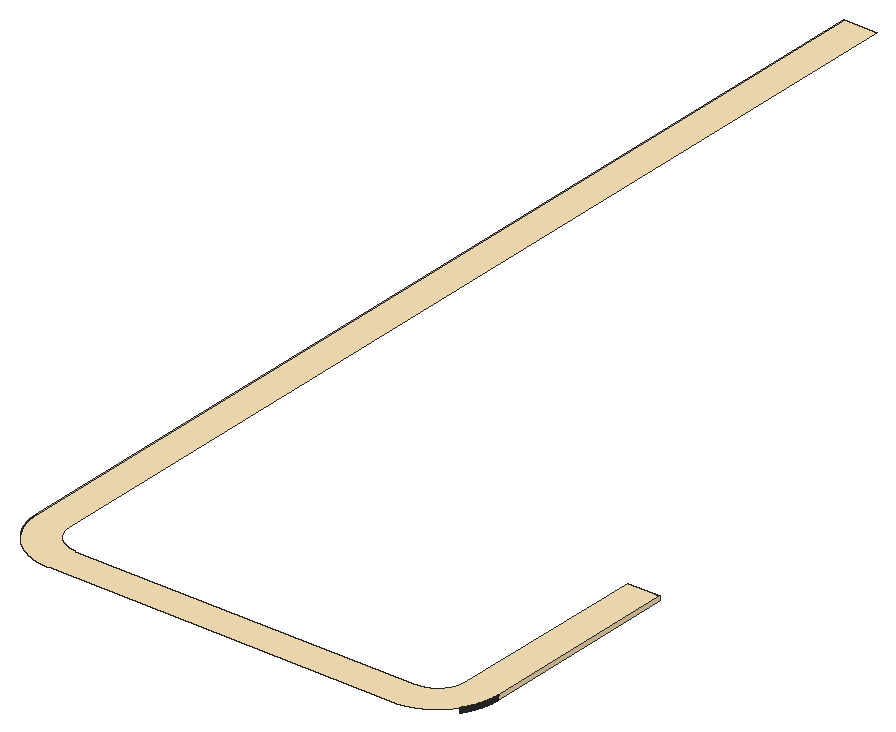
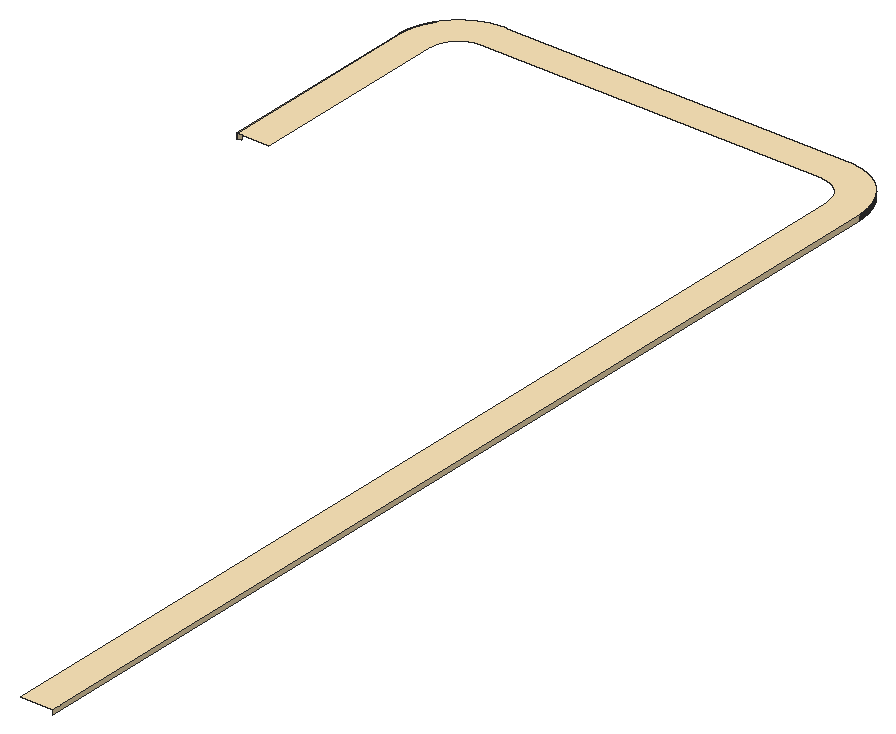
# SketchUp Ruby script. Lengths in inches.
U = 1.inch
M = Sketchup.active_model
def pt(a) = Geom::Point3d.new(a.map { |v| v * U })
def face(e, loops, mat)
  f = e.add_face(loops[0].map { |a| pt(a) })
  loops[1..].each { |l| e.add_face(l.map { |a| pt(a) }).erase! }
  f.material = f.back_material = mat if mat
  f
end
# faces: each face lists its corners as indices into pts; further lists are holes
def faces(e, pts, list, mat = nil) = list.each { |f| face(e, (f[0].is_a?(Array) ? f : [f]).map { |l| l.map { |i| pts[i] } }, mat) }
# xy, xz, yz: faces in a plane at the given z, y or x. An outline is a flat list of corners, or four numbers for a rectangle; further outlines are holes
def ring(l) = l.size == 4 ? [[l[0], l[1]], [l[2], l[1]], [l[2], l[3]], [l[0], l[3]]] : l.each_slice(2).to_a
def flat(e, list, mat, &to3) = list.each { |f| face(e, (f[0].is_a?(Array) ? f : [f]).map { |l| ring(l).map { |u, v| to3.(u, v) } }, mat) }
def xy(e, z, list, mat = nil) = flat(e, list, mat) { |x, y| [x, y, z] }
def xz(e, y, list, mat = nil) = flat(e, list, mat) { |x, z| [x, y, z] }
def yz(e, x, list, mat = nil) = flat(e, list, mat) { |y, z| [x, y, z] }
def lines(e, pts, list) = list.each { |a, b| e.add_line(pt(pts[a]), pt(pts[b])) }
# prism: a flat outline (further loops are holes) pulled along v
def prism(e, loops, v, mat = nil)
  f = face(e, loops, mat); d = Geom::Vector3d.new(v.map { |x| x * U })
  f.pushpull(f.normal.samedirection?(d) ? d.length : -d.length)
end
def box(e, o, s, mat = nil) = prism(e, [[o, [o[0] + s[0], o[1], o[2]], [o[0] + s[0], o[1] + s[1], o[2]], [o[0], o[1] + s[1], o[2]]]], [0, 0, s[2]], mat)
def at(x, y, z, deg = 0) = Geom::Transformation.translation(pt([x, y, z])) * Geom::Transformation.rotation(ORIGIN, Z_AXIS, deg.degrees)
def axes(o, x, y, z) = Geom::Transformation.new([*x, 0, *y, 0, *z, 0, *pt(o).to_a, 1])
def part(name) = M.definitions.add(name)
# library, detail: a bought-in or finely detailed component or shape, given as its bounding box
def library(name, o, s) = part(name).tap { |d| box(d.entities, o, s) }
def detail(e, o, s) = box(e.add_group.entities, o, s)
def put(e, d, t, mat = nil) = e.add_instance(d, t).tap { |i| i.material = mat if mat }
def group(e, t, mat = nil) = e.add_group.tap { |g| g.transformation = t; g.material = mat if mat }.entities
root = M.entities
M.materials.add("1026 AP 7946 SUNNY SIDE UP").color = [254, 231, 186]
xy(root,276,[[[177,213,177.272,213.001,177.545,213.006,177.817,213.013,178.089,213.023,178.361,213.036,178.633,213.051,178.904,213.07,179.176,213.091,179.447,213.115,179.718,213.142,179.988,213.172,180.259,213.205,180.529,213.241,180.798,213.279,181.067,213.32,181.336,213.364,181.604,213.411,181.872,213.461,182.139,213.513,182.406,213.568,182.672,213.626,182.937,213.687,183.202,213.751,183.466,213.817,183.729,213.886,183.992,213.958,184.254,214.032,184.515,214.11,184.775,214.19,185.034,214.273,185.293,214.358,185.551,214.446,185.807,214.537,186.063,214.631,186.318,214.727,186.571,214.826,186.824,214.927,187.075,215.032,187.326,215.138,187.575,215.248,187.823,215.36,188.07,215.474,188.316,215.592,188.561,215.711,188.804,215.834,189.046,215.959,189.286,216.086,189.526,216.216,189.763,216.348,190,216.483,190.235,216.621,190.469,216.761,190.701,216.903,190.931,217.047,191.161,217.195,191.388,217.344,191.614,217.496,191.839,217.65,192.061,217.807,192.282,217.966,192.502,218.127,192.72,218.29,192.936,218.456,193.15,218.624,193.362,218.794,193.573,218.967,193.782,219.141,193.989,219.318,194.194,219.497,194.397,219.678,194.599,219.861,194.798,220.047,194.996,220.234,195.191,220.424,195.385,220.615,195.576,220.809,195.766,221.004,195.953,221.202,196.139,221.401,196.322,221.603,196.503,221.806,196.682,222.011,196.859,222.218,197.033,222.427,197.206,222.638,197.376,222.85,197.544,223.064,197.71,223.28,197.873,223.498,198.034,223.718,198.193,223.939,198.35,224.161,198.504,224.386,198.656,224.612,198.805,224.839,198.953,225.069,199.097,225.299,199.239,225.531,199.379,225.765,199.517,226,199.652,226.237,199.784,226.474,199.914,226.714,200.041,226.954,200.166,227.196,200.289,227.439,200.408,227.684,200.526,227.93,200.64,228.177,200.752,228.425,200.862,228.674,200.968,228.925,201.073,229.176,201.174,229.429,201.273,229.682,201.369,229.937,201.463,230.193,201.554,230.449,201.642,230.707,201.727,230.966,201.81,231.225,201.89,231.485,201.968,231.746,202.042,232.008,202.114,232.271,202.183,232.534,202.249,232.798,202.313,233.063,202.374,233.328,202.432,233.594,202.487,233.861,202.539,234.128,202.589,234.396,202.636,234.664,202.68,234.933,202.721,235.202,202.759,235.471,202.795,235.741,202.828,236.012,202.858,236.282,202.885,236.553,202.909,236.824,202.93,237.096,202.949,237.367,202.964,237.639,202.977,237.911,202.987,238.183,202.994,238.455,202.999,238.728,203,239,203,326,189,326,189,239,188.997,238.749,188.994,238.623,188.989,238.497,188.984,238.372,188.976,238.247,188.968,238.121,188.958,237.996,188.947,237.871,188.934,237.746,188.92,237.621,188.905,237.496,188.889,237.371,188.871,237.247,188.852,237.123,188.832,236.999,188.81,236.875,188.787,236.751,188.763,236.628,188.738,236.505,188.711,236.382,188.683,236.26,188.654,236.138,188.623,236.016,188.591,235.894,188.558,235.773,188.524,235.652,188.488,235.532,188.451,235.412,188.413,235.292,188.373,235.172,188.333,235.054,188.291,234.935,188.247,234.817,188.203,234.7,188.157,234.583,188.11,234.466,188.0625,234.35,188.013,234.234,187.963,234.119,187.911,234.005,187.858,233.891,187.804,233.777,187.749,233.664,187.692,233.552,187.634,233.44,187.576,233.329,187.516,233.219,187.455,233.109,187.392,233,187.329,232.892,187.264,232.784,187.199,232.677,187.132,232.57,187.064,232.464,186.995,232.359,186.925,232.255,186.854,232.151,186.782,232.049,186.634,231.845,186.482,231.645,186.404,231.546,186.326,231.448,186.246,231.351,186.166,231.255,186.084,231.159,186.001,231.064,185.918,230.97,185.833,230.877,185.748,230.785,185.661,230.694,185.574,230.604,185.396,230.426,185.306,230.339,185.215,230.252,185.123,230.167,185.03,230.082,184.936,229.999,184.841,229.916,184.745,229.834,184.649,229.754,184.552,229.674,184.454,229.596,184.355,229.518,184.155,229.366,183.951,229.218,183.849,229.146,183.745,229.075,183.641,229.005,183.536,228.936,183.43,228.868,183.323,228.801,183.216,228.736,183.108,228.671,183,228.608,182.891,228.545,182.781,228.484,182.671,228.424,182.56,228.366,182.448,228.308,182.336,228.251,182.223,228.196,182.109,228.142,181.995,228.089,181.881,228.037,181.766,227.987,181.65,227.9375,181.534,227.89,181.417,227.843,181.3,227.797,181.183,227.753,181.065,227.709,180.946,227.667,180.828,227.627,180.708,227.587,180.588,227.549,180.468,227.512,180.348,227.476,180.227,227.442,180.106,227.409,179.984,227.377,179.862,227.346,179.74,227.317,179.618,227.289,179.495,227.262,179.372,227.237,179.249,227.213,179.125,227.19,179.001,227.168,178.877,227.148,178.753,227.129,178.629,227.111,178.504,227.095,178.379,227.08,178.254,227.066,178.129,227.053,178.004,227.042,177.879,227.032,177.753,227.024,177.628,227.016,177.503,227.011,177.377,227.006,177.251,227.003,177,227,30,227,29.913,227.001,29.749,227.003,29.623,227.006,29.497,227.011,29.372,227.016,29.247,227.024,29.121,227.032,28.996,227.042,28.871,227.053,28.746,227.066,28.621,227.08,28.496,227.095,28.371,227.111,28.247,227.129,28.123,227.148,27.999,227.168,27.875,227.19,27.751,227.213,27.628,227.237,27.505,227.262,27.382,227.289,27.26,227.317,27.138,227.346,27.016,227.377,26.894,227.409,26.773,227.442,26.652,227.476,26.532,227.512,26.412,227.549,26.292,227.587,26.172,227.627,26.054,227.667,25.935,227.709,25.817,227.753,25.7,227.797,25.583,227.843,25.466,227.89,25.35,227.9375,25.234,227.987,25.119,228.037,25.005,228.089,24.891,228.142,24.777,228.196,24.664,228.251,24.552,228.308,24.44,228.366,24.329,228.424,24.219,228.484,24.109,228.545,24,228.608,23.892,228.671,23.784,228.736,23.677,228.801,23.57,228.868,23.464,228.936,23.359,229.005,23.255,229.075,23.151,229.146,23.049,229.218,22.845,229.366,22.645,229.518,22.546,229.596,22.448,229.674,22.351,229.754,22.255,229.834,22.159,229.916,22.064,229.999,21.97,230.082,21.877,230.167,21.785,230.252,21.694,230.339,21.604,230.426,21.426,230.604,21.339,230.694,21.252,230.785,21.167,230.877,21.082,230.97,20.999,231.064,20.916,231.159,20.834,231.255,20.754,231.351,20.674,231.448,20.596,231.546,20.518,231.645,20.366,231.845,20.218,232.049,20.146,232.151,20.075,232.255,20.005,232.359,19.936,232.464,19.868,232.57,19.801,232.677,19.736,232.784,19.671,232.892,19.608,233,19.545,233.109,19.484,233.219,19.424,233.329,19.366,233.44,19.308,233.552,19.251,233.664,19.196,233.777,19.142,233.891,19.089,234.005,19.037,234.119,18.987,234.234,18.9375,234.35,18.89,234.466,18.843,234.583,18.797,234.7,18.753,234.817,18.709,234.935,18.667,235.054,18.627,235.172,18.587,235.292,18.549,235.412,18.512,235.532,18.476,235.652,18.442,235.773,18.409,235.894,18.377,236.016,18.346,236.138,18.317,236.26,18.289,236.382,18.262,236.505,18.237,236.628,18.213,236.751,18.19,236.875,18.168,236.999,18.148,237.123,18.129,237.247,18.111,237.371,18.095,237.496,18.08,237.621,18.066,237.746,18.053,237.871,18.042,237.996,18.032,238.121,18.024,238.247,18.016,238.372,18.011,238.497,18.006,238.623,18.003,238.749,18,239,18,674,4,674,4,238.995,4.001,238.745,4.001,238.728,4.003,238.645,4.005,238.49,4.005,238.472,4.006,238.455,4.008,238.365,4.011,238.234,4.012,238.208,4.013,238.183,4.016,238.094,4.02,237.979,4.022,237.944,4.023,237.911,4.027,237.827,4.031,237.724,4.034,237.68,4.036,237.639,4.04,237.561,4.045,237.469,4.048,237.416,4.051,237.367,4.056,237.296,4.061,237.215,4.066,237.152,4.07,237.096,4.075,237.032,4.08,236.96,4.086,236.888,4.091,236.824,4.096,236.768,4.101,236.706,4.109,236.624,4.115,236.553,4.12,236.505,4.125,236.452,4.135,236.36,4.142,236.282,4.147,236.242,4.151,236.198,4.163,236.095,4.172,236.012,4.176,235.979,4.18,235.944,4.194,235.83,4.205,235.741,4.208,235.717,4.211,235.691,4.229,235.561,4.241,235.471,4.243,235.455,4.245,235.4375,4.267,235.284,4.279,235.202,4.28,235.193,4.281,235.185,4.32,234.933,4.361,234.681,4.363,234.672,4.364,234.664,4.378,234.582,4.408,234.412,4.411,234.396,4.427,234.307,4.451,234.178,4.461,234.128,4.478,234.041,4.5,233.928,4.507,233.893,4.513,233.861,4.53,233.778,4.551,233.678,4.56,233.634,4.568,233.594,4.585,233.518,4.604,233.428,4.616,233.376,4.626,233.328,4.642,233.259,4.66,233.179,4.674,233.118,4.687,233.063,4.702,233,4.718,232.93,4.735,232.861,4.75,232.798,4.764,232.743,4.799,232.603,4.817,232.534,4.829,232.487,4.842,232.435,4.866,232.346,4.886,232.271,4.897,232.231,4.908,232.189,4.935,232.089,4.958,232.008,4.967,231.976,4.976,231.943,5.008,231.832,5.032,231.746,5.039,231.722,5.047,231.697,5.084,231.572,5.11,231.485,5.12,231.453,5.165,231.304,5.19,231.225,5.192,231.217,5.195,231.209,5.273,230.966,5.353,230.723,5.355,230.715,5.358,230.707,5.385,230.629,5.435,230.482,5.441,230.465,5.446,230.449,5.476,230.364,5.52,230.241,5.529,230.216,5.537,230.193,5.568,230.109,5.607,230.001,5.619,229.968,5.631,229.937,5.66,229.858,5.697,229.762,5.712,229.721,5.727,229.682,5.755,229.609,5.788,229.524,5.826,229.429,5.852,229.362,5.883,229.287,5.906,229.229,5.927,229.176,5.952,229.117,5.979,229.05,6.007,228.984,6.032,228.925,6.054,228.872,6.078,228.815,6.11,228.74,6.138,228.674,6.158,228.629,6.179,228.581,6.216,228.497,6.248,228.425,6.265,228.387,6.283,228.347,6.325,228.254,6.36,228.177,6.374,228.147,6.388,228.115,6.437,228.01,6.474,227.93,6.496,227.884,6.553,227.766,6.592,227.684,6.599,227.669,6.607,227.653,6.675,227.514,6.711,227.439,6.715,227.432,6.719,227.424,6.834,227.196,6.951,226.969,6.955,226.962,6.959,226.954,6.997,226.881,7.07,226.744,7.078,226.728,7.086,226.714,7.129,226.634,7.191,226.519,7.204,226.496,7.216,226.474,7.259,226.397,7.315,226.296,7.332,226.265,7.348,226.236,7.39,226.163,7.441,226.074,7.463,226.036,7.483,226,7.523,225.932,7.569,225.853,7.596,225.807,7.621,225.765,7.657,225.704,7.699,225.633,7.731,225.58,7.761,225.531,7.794,225.477,7.831,225.415,7.869,225.354,7.903,225.299,7.933,225.251,7.966,225.198,8.009,225.129,8.047,225.068,8.074,225.027,8.102,224.982,8.152,224.905,8.195,224.839,8.217,224.805,8.241,224.768,8.298,224.682,8.344,224.612,8.362,224.584,8.382,224.555,8.446,224.46,8.496,224.386,8.51,224.365,8.525,224.344,8.599,224.236,8.65,224.161,8.66,224.148,8.67,224.133,8.759,224.006,8.807,223.939,8.817,223.925,8.966,223.718,9.117,223.512,9.127,223.498,9.176,223.432,9.27,223.308,9.29,223.28,9.345,223.209,9.425,223.105,9.441,223.084,9.456,223.064,9.511,222.994,9.582,222.904,9.604,222.876,9.624,222.85,9.677,222.784,9.741,222.704,9.769,222.67,9.794,222.638,9.844,222.577,9.902,222.506,9.936,222.465,9.967,222.427,10.012,222.372,10.065,222.309,10.105,222.262,10.141,222.218,10.183,222.169,10.229,222.114,10.276,222.06,10.318,222.011,10.355,221.968,10.396,221.921,10.45,221.86,10.497,221.806,10.53,221.769,10.565,221.729,10.626,221.661,10.678,221.603,10.706,221.572,10.735,221.539,10.805,221.464,10.861,221.401,10.884,221.377,10.908,221.351,10.986,221.267,11.047,221.202,11.064,221.184,11.172,221.07,11.234,221.004,11.258,220.98,11.366,220.868,11.424,220.809,11.436,220.797,11.615,220.615,11.797,220.436,11.809,220.424,11.868,220.366,11.98,220.258,12.004,220.234,12.07,220.172,12.184,220.064,12.202,220.047,12.267,219.986,12.351,219.908,12.377,219.884,12.401,219.861,12.464,219.805,12.539,219.735,12.572,219.706,12.603,219.678,12.661,219.626,12.729,219.565,12.769,219.53,12.806,219.497,12.86,219.45,12.921,219.396,12.968,219.355,13.011,219.318,13.06,219.276,13.114,219.229,13.169,219.183,13.218,219.141,13.262,219.105,13.309,219.065,13.372,219.012,13.427,218.967,13.465,218.936,13.506,218.902,13.577,218.844,13.638,218.794,13.67,218.769,13.704,218.741,13.784,218.677,13.85,218.624,13.876,218.604,13.904,218.582,13.994,218.511,14.064,218.456,14.084,218.441,14.105,218.425,14.209,218.345,14.28,218.29,14.308,218.27,14.432,218.176,14.498,218.127,14.512,218.117,14.718,217.966,14.925,217.817,14.939,217.807,15.006,217.759,15.133,217.67,15.148,217.66,15.161,217.65,15.236,217.599,15.344,217.525,15.365,217.51,15.386,217.496,15.46,217.446,15.555,217.382,15.584,217.362,15.612,217.344,15.682,217.298,15.768,217.241,15.805,217.217,15.839,217.195,15.905,217.152,15.982,217.102,16.027,217.074,16.068,217.047,16.129,217.009,16.198,216.966,16.251,216.933,16.299,216.903,16.354,216.869,16.415,216.831,16.477,216.794,16.531,216.761,16.58,216.731,16.633,216.699,16.704,216.657,16.765,216.621,16.807,216.596,16.853,216.569,16.932,216.523,17,216.483,17.036,216.463,17.074,216.441,17.163,216.39,17.236,216.348,17.265,216.332,17.296,216.315,17.397,216.259,17.474,216.216,17.496,216.204,17.519,216.191,17.634,216.129,17.714,216.086,17.728,216.078,17.744,216.07,17.881,215.997,17.954,215.959,17.962,215.955,17.969,215.951,18.196,215.834,18.424,215.719,18.432,215.715,18.439,215.711,18.514,215.675,18.653,215.607,18.669,215.599,18.684,215.592,18.766,215.553,18.884,215.496,18.93,215.474,19.01,215.437,19.115,215.388,19.147,215.374,19.177,215.36,19.254,215.325,19.347,215.283,19.387,215.265,19.425,215.248,19.497,215.216,19.581,215.179,19.629,215.158,19.674,215.138,19.74,215.11,19.815,215.078,19.872,215.054,19.925,215.032,19.984,215.007,20.05,214.979,20.117,214.952,20.176,214.927,20.229,214.906,20.287,214.883,20.362,214.852,20.429,214.826,20.524,214.788,20.609,214.755,20.682,214.727,20.721,214.712,20.762,214.697,20.858,214.66,20.937,214.631,20.968,214.619,21.001,214.607,21.109,214.568,21.193,214.537,21.216,214.529,21.241,214.52,21.364,214.476,21.449,214.446,21.465,214.441,21.482,214.435,21.629,214.385,21.707,214.358,21.715,214.355,21.723,214.353,21.966,214.273,22.209,214.195,22.217,214.192,22.225,214.19,22.304,214.165,22.453,214.12,22.485,214.11,22.572,214.084,22.697,214.047,22.722,214.039,22.746,214.032,22.832,214.008,22.943,213.976,22.976,213.967,23.008,213.958,23.089,213.935,23.189,213.908,23.231,213.897,23.271,213.886,23.346,213.866,23.435,213.842,23.487,213.829,23.534,213.817,23.603,213.799,23.743,213.764,23.798,213.75,23.861,213.735,23.93,213.718,24,213.702,24.063,213.687,24.118,213.674,24.179,213.66,24.259,213.642,24.328,213.626,24.376,213.616,24.428,213.604,24.518,213.585,24.594,213.568,24.634,213.56,24.678,213.551,24.778,213.53,24.861,213.513,24.893,213.507,24.928,213.5,25.041,213.478,25.128,213.461,25.178,213.451,25.307,213.427,25.396,213.411,25.412,213.408,25.582,213.378,25.664,213.364,25.672,213.363,25.681,213.361,25.933,213.32,26.185,213.281,26.193,213.28,26.202,213.279,26.284,213.267,26.4375,213.245,26.455,213.243,26.471,213.241,26.561,213.229,26.691,213.211,26.717,213.208,26.741,213.205,26.83,213.194,26.944,213.18,26.979,213.176,27.012,213.172,27.095,213.163,27.198,213.151,27.242,213.147,27.282,213.142,27.36,213.135,27.452,213.125,27.505,213.12,27.553,213.115,27.624,213.109,27.706,213.101,27.768,213.096,27.824,213.091,27.888,213.086,27.96,213.08,28.032,213.075,28.096,213.07,28.152,213.066,28.215,213.061,28.296,213.056,28.367,213.051,28.416,213.048,28.469,213.045,28.561,213.04,28.639,213.036,28.68,213.034,28.724,213.031,28.827,213.027,28.911,213.023,28.944,213.022,28.979,213.02,29.094,213.016,29.183,213.013,29.208,213.012,29.234,213.011,29.365,213.008,29.455,213.006,29.472,213.005,29.49,213.005,29.645,213.003,29.728,213.001,29.75,213.001],[29.764,224.001,29.764,224.002,29.843,224.001]]],"1026 AP 7946 SUNNY SIDE UP")
xz(root,326,[[201,274,203,276]],"1026 AP 7946 SUNNY SIDE UP")
yz(root,4,[[238.995,274,674,276]],"1026 AP 7946 SUNNY SIDE UP")
yz(root,4.001,[[238.728,274,238.736,276],[238.736,274,238.745,276]],"1026 AP 7946 SUNNY SIDE UP")
yz(root,4.005,[[238.472,274,238.49,276]],"1026 AP 7946 SUNNY SIDE UP")
yz(root,203,[[239,274,326,276]],"1026 AP 7946 SUNNY SIDE UP")
p = [[8.67,224.133,276],[8.66,224.148,276],[8.66,224.148,274],[8.67,224.133,274],[8.65,224.161,276],[8.65,224.161,274],
  [8.599,224.236,276],[8.525,224.344,276],[8.525,224.344,274],[8.599,224.236,274],[198.504,224.386,276],[198.35,224.161,276],
  [198.35,224.161,274],[198.504,224.386,274],[8.51,224.365,276],[8.51,224.365,274],[8.496,224.386,276],[8.446,224.46,276],
  [8.446,224.46,274],[8.496,224.386,274],[198.656,224.612,276],[198.656,224.612,274],[8.382,224.555,276],[8.382,224.555,274],
  [8.362,224.584,276],[8.344,224.612,276],[8.344,224.612,274],[8.362,224.584,274],[8.298,224.682,276],[8.298,224.682,274],
  [198.805,224.839,276],[198.805,224.839,274],[8.241,224.768,276],[8.241,224.768,274],[8.217,224.805,276],[8.217,224.805,274],
  [8.195,224.839,276],[8.195,224.839,274],[8.152,224.905,276],[8.152,224.905,274],[198.953,225.069,276],[198.953,225.069,274],
  [8.102,224.982,276],[8.102,224.982,274],[8.074,225.027,276],[8.047,225.068,276],[8.047,225.068,274],[8.074,225.027,274],
  [8.009,225.129,276],[8.009,225.129,274],[7.966,225.198,276],[7.966,225.198,274],[199.097,225.299,276],[199.097,225.299,274],
  [7.933,225.251,276],[7.933,225.251,274],[7.903,225.299,276],[7.903,225.299,274],[7.869,225.354,276],[7.869,225.354,274],
  [199.239,225.531,276],[199.239,225.531,274],[7.831,225.415,276],[7.831,225.415,274],[7.794,225.477,276],[7.794,225.477,274],
  [7.761,225.531,276],[7.731,225.58,276],[7.731,225.58,274],[7.761,225.531,274],[199.379,225.765,276],[199.379,225.765,274],
  [7.699,225.633,276],[7.699,225.633,274],[7.657,225.704,276],[7.657,225.704,274],[7.621,225.765,276],[7.621,225.765,274],
  [7.596,225.807,276],[7.596,225.807,274],[7.569,225.853,276],[7.569,225.853,274],[199.517,226,276],[199.517,226,274],
  [7.523,225.932,276],[7.523,225.932,274],[7.483,226,276],[7.483,226,274],[7.463,226.036,276],[7.441,226.074,276],
  [7.441,226.074,274],[7.463,226.036,274],[199.652,226.237,276],[199.652,226.237,274],[7.39,226.163,276],[7.39,226.163,274],
  [7.348,226.236,276],[7.348,226.236,274],[7.332,226.265,276],[7.332,226.265,274],[199.784,226.474,276],[199.784,226.474,274],
  [7.315,226.296,276],[7.315,226.296,274],[7.259,226.397,276],[7.259,226.397,274],[7.216,226.474,276],[7.216,226.474,274],
  [7.191,226.519,276],[7.129,226.634,276],[7.129,226.634,274],[7.191,226.519,274],[7.204,226.496,276],[7.204,226.496,274],
  [199.914,226.714,276],[199.914,226.714,274],[7.086,226.714,276],[7.086,226.714,274],[7.07,226.744,276],[6.997,226.881,276],
  [6.997,226.881,274],[7.07,226.744,274],[7.078,226.728,276],[7.078,226.728,274],[200.041,226.954,276],[200.041,226.954,274],
  [6.959,226.954,276],[6.959,226.954,274],[6.951,226.969,276],[6.834,227.196,276],[6.834,227.196,274],[6.951,226.969,274],
  [6.955,226.962,276],[6.955,226.962,274],[200.166,227.196,276],[200.166,227.196,274],[6.719,227.424,276],[6.719,227.424,274],
  [200.289,227.439,276],[200.289,227.439,274],[6.715,227.432,276],[6.715,227.432,274],[6.711,227.439,276],[6.711,227.439,274],
  [6.675,227.514,276],[6.675,227.514,274],[200.408,227.684,276],[200.408,227.684,274],[6.607,227.653,276],[6.607,227.653,274],
  [6.599,227.669,276],[6.599,227.669,274],[6.592,227.684,276],[6.592,227.684,274],[6.553,227.766,276],[6.553,227.766,274],
  [200.526,227.93,276],[200.526,227.93,274],[6.496,227.884,276],[6.496,227.884,274],[6.474,227.93,276],[6.437,228.01,276],
  [6.437,228.01,274],[6.474,227.93,274],[6.485,227.907,276],[6.485,227.907,274],[200.64,228.177,276],[200.64,228.177,274],
  [6.388,228.115,276],[6.388,228.115,274],[6.374,228.147,276],[6.374,228.147,274],[6.36,228.177,276],[6.36,228.177,274],
  [6.325,228.254,276],[6.325,228.254,274],[200.752,228.425,276],[200.752,228.425,274],[6.283,228.347,276],[6.283,228.347,274],
  [6.265,228.387,276],[6.265,228.387,274],[6.248,228.425,276],[6.248,228.425,274],[6.216,228.497,276],[6.216,228.497,274],
  [200.862,228.674,276],[200.862,228.674,274],[6.179,228.581,276],[6.179,228.581,274],[6.158,228.629,276],[6.138,228.674,276],
  [6.138,228.674,274],[6.158,228.629,274],[6.11,228.74,276],[6.11,228.74,274],[6.078,228.815,276],[6.078,228.815,274],
  [200.968,228.925,276],[200.968,228.925,274],[6.054,228.872,276],[6.054,228.872,274],[6.032,228.925,276],[6.032,228.925,274],
  [6.007,228.984,276],[6.007,228.984,274],[201.073,229.176,276],[201.073,229.176,274],[5.979,229.05,276],[5.979,229.05,274],
  [5.952,229.117,276],[5.927,229.176,276],[5.927,229.176,274],[5.952,229.117,274],[5.906,229.229,276],[5.906,229.229,274],
  [5.883,229.287,276],[5.883,229.287,274],[201.174,229.429,276],[201.174,229.429,274],[5.852,229.362,276],[5.852,229.362,274],
  [5.826,229.429,276],[5.826,229.429,274],[5.808,229.474,276],[5.808,229.474,274],[201.273,229.682,276],[201.273,229.682,274],
  [5.788,229.524,276],[5.788,229.524,274],[5.755,229.609,276],[5.755,229.609,274],[5.727,229.682,276],[5.727,229.682,274],
  [5.712,229.721,276],[5.712,229.721,274],[5.697,229.762,276],[5.697,229.762,274],[201.369,229.937,276],[201.369,229.937,274],
  [5.66,229.858,276],[5.66,229.858,274],[5.631,229.937,276],[5.631,229.937,274],[5.619,229.968,276],[5.619,229.968,274],
  [201.463,230.193,276],[201.463,230.193,274],[5.607,230.001,276],[5.607,230.001,274],[5.568,230.109,276],[5.568,230.109,274],
  [5.537,230.193,276],[5.537,230.193,274],[5.529,230.216,276],[5.529,230.216,274],[5.52,230.241,276],[5.52,230.241,274],
  [5.476,230.364,276],[5.476,230.364,274],[201.554,230.449,276],[201.554,230.449,274],[5.446,230.449,276],[5.446,230.449,274],
  [5.441,230.465,276],[5.441,230.465,274],[201.642,230.707,276],[201.642,230.707,274],[5.435,230.482,276],[5.435,230.482,274],
  [5.385,230.629,276],[5.385,230.629,274],[5.358,230.707,276],[5.358,230.707,274],[5.353,230.723,276],[5.273,230.966,276],
  [5.273,230.966,274],[5.353,230.723,274],[5.355,230.715,276],[5.355,230.715,274],[201.727,230.966,276],[201.727,230.966,274],
  [5.195,231.209,276],[5.195,231.209,274],[201.81,231.225,276],[201.81,231.225,274],[5.192,231.217,276],[5.192,231.217,274],
  [5.19,231.225,276],[5.19,231.225,274],[5.165,231.304,276],[5.165,231.304,274],[201.89,231.485,276],[201.89,231.485,274],
  [5.12,231.453,276],[5.12,231.453,274],[5.115,231.469,276],[5.115,231.469,274],[5.11,231.485,276],[5.11,231.485,274],
  [5.084,231.572,276],[5.084,231.572,274],[201.968,231.746,276],[201.968,231.746,274],[5.047,231.697,276],[5.047,231.697,274],
  [5.039,231.722,276],[5.039,231.722,274],[5.032,231.746,276],[5.032,231.746,274],[5.008,231.832,276],[5.008,231.832,274],
  [202.042,232.008,276],[202.042,232.008,274],[4.976,231.943,276],[4.976,231.943,274],[4.967,231.976,276],[4.967,231.976,274],
  [4.958,232.008,276],[4.935,232.089,276],[4.935,232.089,274],[4.958,232.008,274],[202.114,232.271,276],[202.114,232.271,274],
  [4.908,232.189,276],[4.908,232.189,274],[4.897,232.231,276],[4.897,232.231,274],[4.886,232.271,276],[4.886,232.271,274],
  [4.866,232.346,276],[4.842,232.435,276],[4.842,232.435,274],[4.866,232.346,274],[202.183,232.534,276],[202.183,232.534,274],
  [4.829,232.487,276],[4.829,232.487,274],[4.817,232.534,276],[4.817,232.534,274],[4.799,232.603,276],[4.799,232.603,274],
  [202.249,232.798,276],[202.249,232.798,274],[4.779,232.683,276],[4.779,232.683,274],[4.764,232.743,276],[4.764,232.743,274],
  [4.75,232.798,276],[4.75,232.798,274],[4.735,232.861,276],[4.735,232.861,274],[202.313,233.063,276],[202.313,233.063,274],
  [4.718,232.93,276],[4.718,232.93,274],[4.702,233,276],[4.702,233,274],[4.687,233.063,276],[4.687,233.063,274],
  [4.674,233.118,276],[4.674,233.118,274],[4.66,233.179,276],[4.66,233.179,274],[202.374,233.328,276],[202.374,233.328,274],
  [4.642,233.259,276],[4.642,233.259,274],[4.626,233.328,276],[4.626,233.328,274],[4.616,233.376,276],[4.616,233.376,274],
  [202.432,233.594,276],[202.432,233.594,274],[4.604,233.428,276],[4.604,233.428,274],[4.585,233.518,276],[4.585,233.518,274],
  [4.568,233.594,276],[4.568,233.594,274],[4.56,233.634,276],[4.56,233.634,274],[4.551,233.678,276],[4.551,233.678,274],
  [202.487,233.861,276],[202.487,233.861,274],[4.53,233.778,276],[4.53,233.778,274],[4.513,233.861,276],[4.513,233.861,274],
  [4.507,233.893,276],[4.507,233.893,274],[4.5,233.928,276],[4.5,233.928,274],[4.478,234.041,276],[4.478,234.041,274],
  [202.539,234.128,276],[202.539,234.128,274],[4.461,234.128,276],[4.461,234.128,274],[4.456,234.153,276],[4.456,234.153,274],
  [202.589,234.396,276],[202.589,234.396,274],[4.451,234.178,276],[4.427,234.307,276],[4.427,234.307,274],[4.451,234.178,274],
  [4.411,234.396,276],[4.411,234.396,274],[4.408,234.412,276],[4.408,234.412,274],[4.405,234.429,276],[4.405,234.429,274],
  [4.378,234.582,276],[4.378,234.582,274],[202.636,234.664,276],[202.636,234.664,274],[4.364,234.664,276],[4.364,234.664,274],
  [4.361,234.681,276],[4.32,234.933,276],[4.32,234.933,274],[4.361,234.681,274],[4.363,234.672,276],[4.363,234.672,274],
  [202.68,234.933,276],[202.68,234.933,274],[4.281,235.185,276],[4.281,235.185,274],[202.721,235.202,276],[202.721,235.202,274],
  [4.28,235.193,276],[4.28,235.193,274],[4.279,235.202,276],[4.279,235.202,274],[4.267,235.284,276],[4.267,235.284,274],
  [202.759,235.471,276],[202.759,235.471,274],[4.245,235.4375,276],[4.245,235.4375,274],[4.243,235.455,276],[4.243,235.455,274],
  [4.241,235.471,276],[4.241,235.471,274],[4.229,235.561,276],[4.229,235.561,274],[202.795,235.741,276],[202.795,235.741,274],
  [4.211,235.691,276],[4.211,235.691,274],[4.208,235.717,276],[4.208,235.717,274],[4.205,235.741,276],[4.205,235.741,274],
  [4.194,235.83,276],[4.194,235.83,274],[202.828,236.012,276],[202.828,236.012,274],[4.18,235.944,276],[4.18,235.944,274],
  [4.176,235.979,276],[4.176,235.979,274],[4.172,236.012,276],[4.172,236.012,274],[4.163,236.095,276],[4.163,236.095,274],
  [202.858,236.282,276],[202.858,236.282,274],[4.151,236.198,276],[4.151,236.198,274],[4.147,236.242,276],[4.147,236.242,274],
  [4.142,236.282,276],[4.142,236.282,274],[4.135,236.36,276],[4.135,236.36,274],[202.885,236.553,276],[202.885,236.553,274],
  [4.125,236.452,276],[4.125,236.452,274],[4.12,236.505,276],[4.12,236.505,274],[4.115,236.553,276],[4.115,236.553,274],
  [4.109,236.624,276],[4.109,236.624,274],[4.101,236.706,276],[4.101,236.706,274],[202.909,236.824,276],[202.909,236.824,274],
  [4.096,236.768,276],[4.096,236.768,274],[4.091,236.824,276],[4.091,236.824,274],[4.086,236.888,276],[4.086,236.888,274],
  [202.93,237.096,276],[202.93,237.096,274],[4.08,236.96,276],[4.08,236.96,274],[4.075,237.032,276],[4.075,237.032,274],
  [4.07,237.096,276],[4.07,237.096,274],[4.066,237.152,276],[4.066,237.152,274],[202.949,237.367,276],[202.949,237.367,274],
  [4.061,237.215,276],[4.061,237.215,274],[4.056,237.296,276],[4.056,237.296,274],[4.051,237.367,276],[4.051,237.367,274],
  [4.048,237.416,276],[4.048,237.416,274],[4.045,237.469,276],[4.045,237.469,274],[202.964,237.639,276],[202.964,237.639,274],
  [4.04,237.561,276],[4.04,237.561,274],[4.036,237.639,276],[4.036,237.639,274],[4.034,237.68,276],[4.034,237.68,274],
  [202.977,237.911,276],[202.977,237.911,274],[4.031,237.724,276],[4.031,237.724,274],[4.027,237.827,276],[4.027,237.827,274],
  [4.023,237.911,276],[4.023,237.911,274],[4.022,237.944,276],[4.022,237.944,274],[4.02,237.979,276],[4.02,237.979,274],
  [202.987,238.183,276],[202.987,238.183,274],[4.016,238.094,276],[4.016,238.094,274],[4.013,238.183,276],[4.013,238.183,274],
  [4.012,238.208,276],[4.012,238.208,274],[4.011,238.234,276],[4.011,238.234,274],[4.008,238.365,276],[4.008,238.365,274],
  [202.994,238.455,276],[202.994,238.455,274],[4.006,238.455,276],[4.006,238.455,274],[4.005,238.472,276],[4.005,238.472,274],
  [4.005,238.49,276],[4.003,238.645,276],[4.003,238.645,274],[4.005,238.49,274],[202.999,238.728,276],[202.999,238.728,274],
  [4.001,238.728,276],[4.001,238.728,274],[4.001,238.745,276],[4,238.995,276],[4,238.995,274],[4.001,238.745,274],
  [203,239,276],[203,239,274],[201,239,274],[201,239,276],[6,239,274],[6,239,276]]
faces(root,p,[[0,1,2,3],[1,4,5,2],[6,7,8,9],[4,6,9,5],[10,11,12,13],[7,14,15,8],[16,17,18,19],[14,16,19,15],
  [20,10,13,21],[17,22,23,18],[24,25,26,27],[25,28,29,26],[22,24,27,23],[30,20,21,31],[28,32,33,29],[32,34,35,33],
  [34,36,37,35],[36,38,39,37],[40,30,31,41],[38,42,43,39],[44,45,46,47],[42,44,47,43],[45,48,49,46],[48,50,51,49],
  [52,40,41,53],[50,54,55,51],[54,56,57,55],[56,58,59,57],[60,52,53,61],[58,62,63,59],[62,64,65,63],[66,67,68,69],
  [64,66,69,65],[70,60,61,71],[67,72,73,68],[72,74,75,73],[74,76,77,75],[76,78,79,77],[78,80,81,79],[82,70,71,83],
  [80,84,85,81],[84,86,87,85],[88,89,90,91],[86,88,91,87],[92,82,83,93],[89,94,95,90],[94,96,97,95],[96,98,99,97],
  [100,92,93,101],[98,102,103,99],[102,104,105,103],[104,106,107,105],[108,109,110,111],[106,112,113,107],[112,108,111,113],[114,100,101,115],
  [109,116,117,110],[118,119,120,121],[116,122,123,117],[122,118,121,123],[124,114,115,125],[119,126,127,120],[128,129,130,131],[126,132,133,127],
  [132,128,131,133],[134,124,125,135],[129,136,137,130],[138,134,135,139],[136,140,141,137],[140,142,143,141],[142,144,145,143],[146,138,139,147],
  [144,148,149,145],[148,150,151,149],[150,152,153,151],[152,154,155,153],[156,146,147,157],[154,158,159,155],[160,161,162,163],[158,164,165,159],
  [164,160,163,165],[166,156,157,167],[161,168,169,162],[168,170,171,169],[170,172,173,171],[172,174,175,173],[176,166,167,177],[174,178,179,175],
  [178,180,181,179],[180,182,183,181],[182,184,185,183],[186,176,177,187],[184,188,189,185],[190,191,192,193],[188,190,193,189],[191,194,195,192],
  [194,196,197,195],[198,186,187,199],[196,200,201,197],[200,202,203,201],[202,204,205,203],[206,198,199,207],[204,208,209,205],[210,211,212,213],
  [208,210,213,209],[211,214,215,212],[214,216,217,215],[218,206,207,219],[216,220,221,217],[220,222,223,221],[222,224,225,223],[226,218,219,227],
  [224,228,229,225],[228,230,231,229],[230,232,233,231],[232,234,235,233],[234,236,237,235],[238,226,227,239],[236,240,241,237],[240,242,243,241],
  [242,244,245,243],[246,238,239,247],[244,248,249,245],[248,250,251,249],[250,252,253,251],[252,254,255,253],[254,256,257,255],[256,258,259,257],
  [260,246,247,261],[258,262,263,259],[262,264,265,263],[266,260,261,267],[264,268,269,265],[268,270,271,269],[270,272,273,271],[274,275,276,277],
  [272,278,279,273],[278,274,277,279],[280,266,267,281],[275,282,283,276],[284,280,281,285],[282,286,287,283],[286,288,289,287],[288,290,291,289],
  [292,284,285,293],[290,294,295,291],[294,296,297,295],[296,298,299,297],[298,300,301,299],[302,292,293,303],[300,304,305,301],[304,306,307,305],
  [306,308,309,307],[308,310,311,309],[312,302,303,313],[310,314,315,311],[314,316,317,315],[318,319,320,321],[316,318,321,317],[322,312,313,323],
  [319,324,325,320],[324,326,327,325],[326,328,329,327],[330,331,332,333],[328,330,333,329],[334,322,323,335],[331,336,337,332],[336,338,339,337],
  [338,340,341,339],[342,334,335,343],[340,344,345,341],[344,346,347,345],[346,348,349,347],[348,350,351,349],[352,342,343,353],[350,354,355,351],
  [354,356,357,355],[356,358,359,357],[358,360,361,359],[360,362,363,361],[364,352,353,365],[362,366,367,363],[366,368,369,367],[368,370,371,369],
  [372,364,365,373],[370,374,375,371],[374,376,377,375],[376,378,379,377],[378,380,381,379],[380,382,383,381],[384,372,373,385],[382,386,387,383],
  [386,388,389,387],[388,390,391,389],[390,392,393,391],[392,394,395,393],[396,384,385,397],[394,398,399,395],[398,400,401,399],[402,396,397,403],
  [404,405,406,407],[400,404,407,401],[405,408,409,406],[408,410,411,409],[410,412,413,411],[412,414,415,413],[416,402,403,417],[414,418,419,415],
  [420,421,422,423],[418,424,425,419],[424,420,423,425],[426,416,417,427],[421,428,429,422],[430,426,427,431],[428,432,433,429],[432,434,435,433],
  [434,436,437,435],[438,430,431,439],[436,440,441,437],[440,442,443,441],[442,444,445,443],[444,446,447,445],[448,438,439,449],[446,450,451,447],
  [450,452,453,451],[452,454,455,453],[454,456,457,455],[458,448,449,459],[456,460,461,457],[460,462,463,461],[462,464,465,463],[464,466,467,465],
  [468,458,459,469],[466,470,471,467],[470,472,473,471],[472,474,475,473],[474,476,477,475],[478,468,469,479],[476,480,481,477],[480,482,483,481],
  [482,484,485,483],[484,486,487,485],[486,488,489,487],[490,478,479,491],[488,492,493,489],[492,494,495,493],[494,496,497,495],[498,490,491,499],
  [496,500,501,497],[500,502,503,501],[502,504,505,503],[504,506,507,505],[508,498,499,509],[506,510,511,507],[510,512,513,511],[512,514,515,513],
  [514,516,517,515],[516,518,519,517],[520,508,509,521],[518,522,523,519],[522,524,525,523],[524,526,527,525],[528,520,521,529],[526,530,531,527],
  [530,532,533,531],[532,534,535,533],[534,536,537,535],[536,538,539,537],[540,528,529,541],[538,542,543,539],[542,544,545,543],[544,546,547,545],
  [546,548,549,547],[548,550,551,549],[552,540,541,553],[550,554,555,551],[554,556,557,555],[558,559,560,561],[562,552,553,563],[559,564,565,560],
  [566,567,568,569],[570,562,563,571]],"1026 AP 7946 SUNNY SIDE UP")
lines(root,p,[[572,573],[574,575]])
